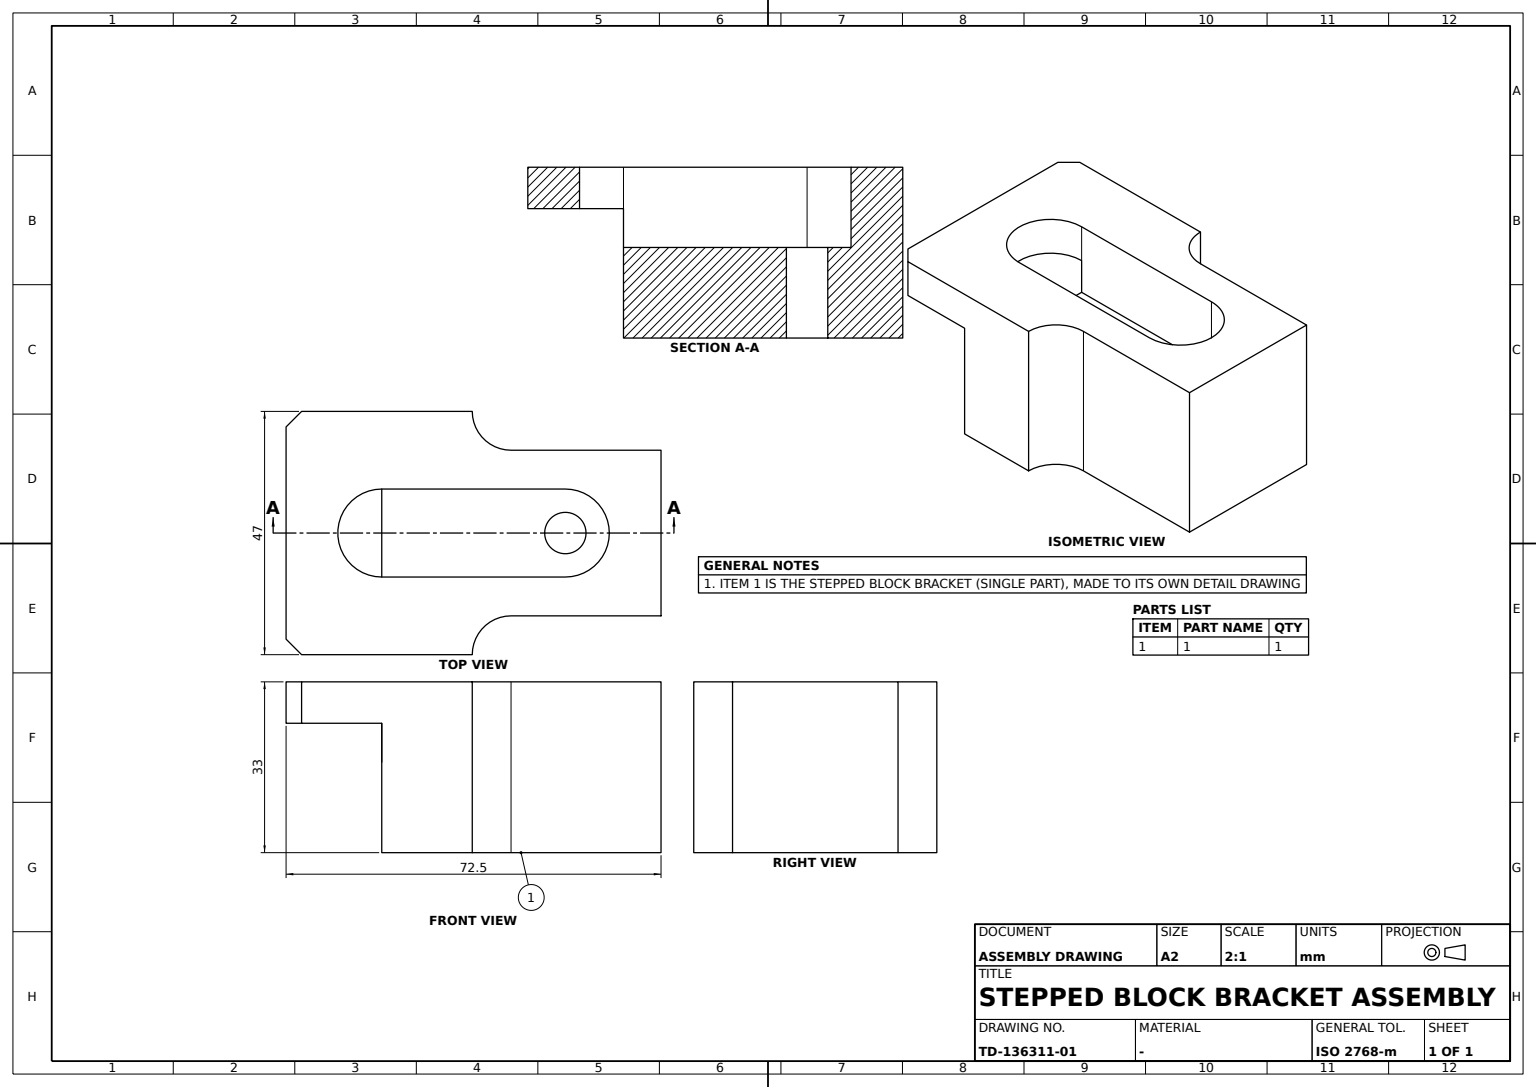
ISO-10303-21;
HEADER;
FILE_DESCRIPTION((''),'2;1');
FILE_NAME('','',(''),(''),'','','');
FILE_SCHEMA(('AUTOMOTIVE_DESIGN'));
ENDSEC;
DATA;
#1=APPLICATION_CONTEXT('');
#2=PRODUCT_CONTEXT('',#1,'mechanical');
#3=PRODUCT('','','',(#2));
#4=PRODUCT_DEFINITION_FORMATION('','',#3);
#5=PRODUCT_DEFINITION_CONTEXT('',#1,'design');
#6=PRODUCT_DEFINITION('','',#4,#5);
#7=PRODUCT_DEFINITION_SHAPE('','',#6);
#8=(LENGTH_UNIT()NAMED_UNIT(*)SI_UNIT(.MILLI.,.METRE.));
#9=(NAMED_UNIT(*)PLANE_ANGLE_UNIT()SI_UNIT($,.RADIAN.));
#10=(NAMED_UNIT(*)SI_UNIT($,.STERADIAN.)SOLID_ANGLE_UNIT());
#11=UNCERTAINTY_MEASURE_WITH_UNIT(LENGTH_MEASURE(1.E-05),#8,'distance_accuracy_value','');
#12=(GEOMETRIC_REPRESENTATION_CONTEXT(3)GLOBAL_UNCERTAINTY_ASSIGNED_CONTEXT((#11))GLOBAL_UNIT_ASSIGNED_CONTEXT((#8,#9,#10))REPRESENTATION_CONTEXT('',''));
#13=CARTESIAN_POINT('',(21.75,0.,17.5));
#14=VERTEX_POINT('',#13);
#15=CARTESIAN_POINT('',(13.75,0.,17.5));
#16=VERTEX_POINT('',#15);
#17=CARTESIAN_POINT('',(17.75,0.,17.5));
#18=DIRECTION('',(0.,0.,1.));
#19=DIRECTION('',(1.,0.,0.));
#20=AXIS2_PLACEMENT_3D('',#17,#18,#19);
#21=CIRCLE('',#20,4.);
#22=EDGE_CURVE('',#14,#16,#21,.T.);
#23=ORIENTED_EDGE('',*,*,#22,.T.);
#24=CARTESIAN_POINT('',(13.75,0.,0.));
#25=VERTEX_POINT('',#24);
#26=CARTESIAN_POINT('',(13.75,0.,-54982.5));
#27=VECTOR('',#18,1000.);
#28=LINE('',#26,#27);
#29=EDGE_CURVE('',#25,#16,#28,.T.);
#30=ORIENTED_EDGE('',*,*,#29,.F.);
#31=CARTESIAN_POINT('',(21.75,0.,0.));
#32=VERTEX_POINT('',#31);
#33=CARTESIAN_POINT('',(17.75,0.,0.));
#34=AXIS2_PLACEMENT_3D('',#33,#18,#19);
#35=CIRCLE('',#34,4.);
#36=EDGE_CURVE('',#32,#25,#35,.T.);
#37=ORIENTED_EDGE('',*,*,#36,.F.);
#38=CARTESIAN_POINT('',(21.75,0.,-54982.5));
#39=LINE('',#38,#27);
#40=EDGE_CURVE('',#32,#14,#39,.T.);
#41=ORIENTED_EDGE('',*,*,#40,.T.);
#42=EDGE_LOOP('',(#23,#30,#37,#41));
#43=FACE_OUTER_BOUND('',#42,.T.);
#44=CARTESIAN_POINT('',(17.75,0.,-54982.5));
#45=AXIS2_PLACEMENT_3D('',#44,#18,#19);
#46=CYLINDRICAL_SURFACE('',#45,4.);
#47=ADVANCED_FACE('',(#43),#46,.F.);
#48=CARTESIAN_POINT('',(-17.75,-8.5,33.));
#49=VERTEX_POINT('',#48);
#50=CARTESIAN_POINT('',(17.75,-8.5,33.));
#51=VERTEX_POINT('',#50);
#52=VECTOR('',#19,1000.);
#53=LINE('',#48,#52);
#54=EDGE_CURVE('',#49,#51,#53,.T.);
#55=ORIENTED_EDGE('',*,*,#54,.F.);
#56=CARTESIAN_POINT('',(-17.75,8.5,33.));
#57=VERTEX_POINT('',#56);
#58=CARTESIAN_POINT('',(-17.75,0.,33.));
#59=AXIS2_PLACEMENT_3D('',#58,#18,#19);
#60=CIRCLE('',#59,8.5);
#61=EDGE_CURVE('',#57,#49,#60,.T.);
#62=ORIENTED_EDGE('',*,*,#61,.F.);
#63=CARTESIAN_POINT('',(17.75,8.5,33.));
#64=VERTEX_POINT('',#63);
#65=DIRECTION('',(-1.,0.,0.));
#66=VECTOR('',#65,1000.);
#67=LINE('',#63,#66);
#68=EDGE_CURVE('',#64,#57,#67,.T.);
#69=ORIENTED_EDGE('',*,*,#68,.F.);
#70=CARTESIAN_POINT('',(26.25,0.,33.));
#71=VERTEX_POINT('',#70);
#72=CARTESIAN_POINT('',(17.75,0.,33.));
#73=AXIS2_PLACEMENT_3D('',#72,#18,#19);
#74=CIRCLE('',#73,8.5);
#75=EDGE_CURVE('',#71,#64,#74,.T.);
#76=ORIENTED_EDGE('',*,*,#75,.F.);
#77=EDGE_CURVE('',#51,#71,#74,.T.);
#78=ORIENTED_EDGE('',*,*,#77,.F.);
#79=EDGE_LOOP('',(#55,#62,#69,#76,#78));
#80=FACE_BOUND('',#79,.T.);
#81=CARTESIAN_POINT('',(36.25,-16.,33.));
#82=VERTEX_POINT('',#81);
#83=CARTESIAN_POINT('',(7.25,-16.,33.));
#84=VERTEX_POINT('',#83);
#85=LINE('',#81,#66);
#86=EDGE_CURVE('',#82,#84,#85,.T.);
#87=ORIENTED_EDGE('',*,*,#86,.F.);
#88=CARTESIAN_POINT('',(36.25,16.,33.));
#89=VERTEX_POINT('',#88);
#90=CARTESIAN_POINT('',(36.25,-23.5,33.));
#91=DIRECTION('',(0.,1.,0.));
#92=VECTOR('',#91,1000.);
#93=LINE('',#90,#92);
#94=EDGE_CURVE('',#82,#89,#93,.T.);
#95=ORIENTED_EDGE('',*,*,#94,.T.);
#96=CARTESIAN_POINT('',(7.25,16.,33.));
#97=VERTEX_POINT('',#96);
#98=CARTESIAN_POINT('',(-0.25,16.,33.));
#99=LINE('',#98,#52);
#100=EDGE_CURVE('',#97,#89,#99,.T.);
#101=ORIENTED_EDGE('',*,*,#100,.F.);
#102=CARTESIAN_POINT('',(-0.25,23.5,33.));
#103=VERTEX_POINT('',#102);
#104=CARTESIAN_POINT('',(7.25,23.5,33.));
#105=DIRECTION('',(0.,0.,-1.));
#106=AXIS2_PLACEMENT_3D('',#104,#105,#19);
#107=CIRCLE('',#106,7.5);
#108=EDGE_CURVE('',#97,#103,#107,.T.);
#109=ORIENTED_EDGE('',*,*,#108,.T.);
#110=CARTESIAN_POINT('',(-33.25,23.5,33.));
#111=VERTEX_POINT('',#110);
#112=CARTESIAN_POINT('',(36.25,23.5,33.));
#113=LINE('',#112,#66);
#114=EDGE_CURVE('',#103,#111,#113,.T.);
#115=ORIENTED_EDGE('',*,*,#114,.T.);
#116=CARTESIAN_POINT('',(-36.25,20.5,33.));
#117=VERTEX_POINT('',#116);
#118=DIRECTION('',(-0.707106781,-0.707106781,0.));
#119=VECTOR('',#118,1000.);
#120=LINE('',#110,#119);
#121=EDGE_CURVE('',#111,#117,#120,.T.);
#122=ORIENTED_EDGE('',*,*,#121,.T.);
#123=CARTESIAN_POINT('',(-36.25,-20.5,33.));
#124=VERTEX_POINT('',#123);
#125=DIRECTION('',(0.,-1.,0.));
#126=VECTOR('',#125,1000.);
#127=LINE('',#116,#126);
#128=EDGE_CURVE('',#117,#124,#127,.T.);
#129=ORIENTED_EDGE('',*,*,#128,.T.);
#130=CARTESIAN_POINT('',(-33.25,-23.5,33.));
#131=VERTEX_POINT('',#130);
#132=DIRECTION('',(0.707106781,-0.707106781,0.));
#133=VECTOR('',#132,1000.);
#134=LINE('',#123,#133);
#135=EDGE_CURVE('',#124,#131,#134,.T.);
#136=ORIENTED_EDGE('',*,*,#135,.T.);
#137=CARTESIAN_POINT('',(-0.25,-23.5,33.));
#138=VERTEX_POINT('',#137);
#139=LINE('',#130,#52);
#140=EDGE_CURVE('',#131,#138,#139,.T.);
#141=ORIENTED_EDGE('',*,*,#140,.T.);
#142=CARTESIAN_POINT('',(7.25,-23.5,33.));
#143=AXIS2_PLACEMENT_3D('',#142,#105,#19);
#144=CIRCLE('',#143,7.5);
#145=EDGE_CURVE('',#138,#84,#144,.T.);
#146=ORIENTED_EDGE('',*,*,#145,.T.);
#147=EDGE_LOOP('',(#87,#95,#101,#109,#115,#122,#129,#136,#141,#146));
#148=FACE_OUTER_BOUND('',#147,.T.);
#149=CARTESIAN_POINT('',(0.,0.,33.));
#150=AXIS2_PLACEMENT_3D('',#149,#18,#19);
#151=PLANE('',#150);
#152=ADVANCED_FACE('',(#80,#148),#151,.T.);
#153=CARTESIAN_POINT('',(-17.75,-8.5,25.));
#154=VERTEX_POINT('',#153);
#155=CARTESIAN_POINT('',(-17.75,-8.5,17.5));
#156=VECTOR('',#105,1000.);
#157=LINE('',#155,#156);
#158=EDGE_CURVE('',#49,#154,#157,.T.);
#159=ORIENTED_EDGE('',*,*,#158,.T.);
#160=CARTESIAN_POINT('',(-17.75,8.5,25.));
#161=VERTEX_POINT('',#160);
#162=CARTESIAN_POINT('',(-17.75,0.,25.));
#163=AXIS2_PLACEMENT_3D('',#162,#18,#19);
#164=CIRCLE('',#163,8.5);
#165=EDGE_CURVE('',#161,#154,#164,.T.);
#166=ORIENTED_EDGE('',*,*,#165,.F.);
#167=CARTESIAN_POINT('',(-17.75,8.5,17.5));
#168=LINE('',#167,#156);
#169=EDGE_CURVE('',#57,#161,#168,.T.);
#170=ORIENTED_EDGE('',*,*,#169,.F.);
#171=ORIENTED_EDGE('',*,*,#61,.T.);
#172=EDGE_LOOP('',(#159,#166,#170,#171));
#173=FACE_OUTER_BOUND('',#172,.T.);
#174=CARTESIAN_POINT('',(-17.75,0.,17.5));
#175=AXIS2_PLACEMENT_3D('',#174,#18,#19);
#176=CYLINDRICAL_SURFACE('',#175,8.5);
#177=ADVANCED_FACE('',(#173),#176,.F.);
#178=CARTESIAN_POINT('',(-36.25,-20.5,25.));
#179=VERTEX_POINT('',#178);
#180=LINE('',#123,#156);
#181=EDGE_CURVE('',#124,#179,#180,.T.);
#182=ORIENTED_EDGE('',*,*,#181,.F.);
#183=ORIENTED_EDGE('',*,*,#128,.F.);
#184=CARTESIAN_POINT('',(-36.25,20.5,25.));
#185=VERTEX_POINT('',#184);
#186=LINE('',#116,#156);
#187=EDGE_CURVE('',#117,#185,#186,.T.);
#188=ORIENTED_EDGE('',*,*,#187,.T.);
#189=CARTESIAN_POINT('',(-36.25,54976.5,25.));
#190=LINE('',#189,#126);
#191=EDGE_CURVE('',#185,#179,#190,.T.);
#192=ORIENTED_EDGE('',*,*,#191,.T.);
#193=EDGE_LOOP('',(#182,#183,#188,#192));
#194=FACE_OUTER_BOUND('',#193,.T.);
#195=AXIS2_PLACEMENT_3D('',#116,#19,#91);
#196=PLANE('',#195);
#197=ADVANCED_FACE('',(#194),#196,.F.);
#198=CARTESIAN_POINT('',(-0.25,-23.5,0.));
#199=VERTEX_POINT('',#198);
#200=LINE('',#198,#27);
#201=EDGE_CURVE('',#199,#138,#200,.T.);
#202=ORIENTED_EDGE('',*,*,#201,.T.);
#203=ORIENTED_EDGE('',*,*,#140,.F.);
#204=CARTESIAN_POINT('',(-33.25,-23.5,25.));
#205=VERTEX_POINT('',#204);
#206=LINE('',#130,#156);
#207=EDGE_CURVE('',#131,#205,#206,.T.);
#208=ORIENTED_EDGE('',*,*,#207,.T.);
#209=CARTESIAN_POINT('',(-17.75,-23.5,25.));
#210=VERTEX_POINT('',#209);
#211=LINE('',#209,#66);
#212=EDGE_CURVE('',#210,#205,#211,.T.);
#213=ORIENTED_EDGE('',*,*,#212,.F.);
#214=CARTESIAN_POINT('',(-17.75,-23.5,0.));
#215=VERTEX_POINT('',#214);
#216=LINE('',#214,#27);
#217=EDGE_CURVE('',#215,#210,#216,.T.);
#218=ORIENTED_EDGE('',*,*,#217,.F.);
#219=CARTESIAN_POINT('',(-33.25,-23.5,0.));
#220=LINE('',#219,#52);
#221=EDGE_CURVE('',#215,#199,#220,.T.);
#222=ORIENTED_EDGE('',*,*,#221,.T.);
#223=EDGE_LOOP('',(#202,#203,#208,#213,#218,#222));
#224=FACE_OUTER_BOUND('',#223,.T.);
#225=AXIS2_PLACEMENT_3D('',#130,#91,#18);
#226=PLANE('',#225);
#227=ADVANCED_FACE('',(#224),#226,.F.);
#228=ORIENTED_EDGE('',*,*,#121,.F.);
#229=CARTESIAN_POINT('',(-33.25,23.5,25.));
#230=VERTEX_POINT('',#229);
#231=LINE('',#110,#156);
#232=EDGE_CURVE('',#111,#230,#231,.T.);
#233=ORIENTED_EDGE('',*,*,#232,.T.);
#234=LINE('',#229,#119);
#235=EDGE_CURVE('',#230,#185,#234,.T.);
#236=ORIENTED_EDGE('',*,*,#235,.T.);
#237=ORIENTED_EDGE('',*,*,#187,.F.);
#238=EDGE_LOOP('',(#228,#233,#236,#237));
#239=FACE_OUTER_BOUND('',#238,.T.);
#240=DIRECTION('',(0.707106781,0.707106781,0.));
#241=AXIS2_PLACEMENT_3D('',#110,#132,#240);
#242=PLANE('',#241);
#243=ADVANCED_FACE('',(#239),#242,.F.);
#244=CARTESIAN_POINT('',(36.25,16.,0.));
#245=VERTEX_POINT('',#244);
#246=CARTESIAN_POINT('',(36.25,16.,-54967.));
#247=LINE('',#246,#27);
#248=EDGE_CURVE('',#245,#89,#247,.T.);
#249=ORIENTED_EDGE('',*,*,#248,.T.);
#250=ORIENTED_EDGE('',*,*,#94,.F.);
#251=CARTESIAN_POINT('',(36.25,-16.,0.));
#252=VERTEX_POINT('',#251);
#253=LINE('',#251,#27);
#254=EDGE_CURVE('',#252,#82,#253,.T.);
#255=ORIENTED_EDGE('',*,*,#254,.F.);
#256=CARTESIAN_POINT('',(36.25,-23.5,0.));
#257=LINE('',#256,#92);
#258=EDGE_CURVE('',#252,#245,#257,.T.);
#259=ORIENTED_EDGE('',*,*,#258,.T.);
#260=EDGE_LOOP('',(#249,#250,#255,#259));
#261=FACE_OUTER_BOUND('',#260,.T.);
#262=AXIS2_PLACEMENT_3D('',#90,#65,#125);
#263=PLANE('',#262);
#264=ADVANCED_FACE('',(#261),#263,.F.);
#265=CARTESIAN_POINT('',(7.25,-16.,0.));
#266=VERTEX_POINT('',#265);
#267=CARTESIAN_POINT('',(7.25,-23.5,0.));
#268=AXIS2_PLACEMENT_3D('',#267,#18,#19);
#269=CIRCLE('',#268,7.5);
#270=EDGE_CURVE('',#266,#199,#269,.T.);
#271=ORIENTED_EDGE('',*,*,#270,.F.);
#272=LINE('',#265,#156);
#273=EDGE_CURVE('',#84,#266,#272,.T.);
#274=ORIENTED_EDGE('',*,*,#273,.F.);
#275=ORIENTED_EDGE('',*,*,#145,.F.);
#276=ORIENTED_EDGE('',*,*,#201,.F.);
#277=EDGE_LOOP('',(#271,#274,#275,#276));
#278=FACE_OUTER_BOUND('',#277,.T.);
#279=CYLINDRICAL_SURFACE('',#268,7.5);
#280=ADVANCED_FACE('',(#278),#279,.F.);
#281=ORIENTED_EDGE('',*,*,#77,.T.);
#282=CARTESIAN_POINT('',(26.25,0.,17.5));
#283=VERTEX_POINT('',#282);
#284=LINE('',#282,#27);
#285=EDGE_CURVE('',#283,#71,#284,.T.);
#286=ORIENTED_EDGE('',*,*,#285,.F.);
#287=CARTESIAN_POINT('',(17.75,-8.5,17.5));
#288=VERTEX_POINT('',#287);
#289=AXIS2_PLACEMENT_3D('',#17,#105,#19);
#290=CIRCLE('',#289,8.5);
#291=EDGE_CURVE('',#283,#288,#290,.T.);
#292=ORIENTED_EDGE('',*,*,#291,.T.);
#293=LINE('',#287,#156);
#294=EDGE_CURVE('',#51,#288,#293,.T.);
#295=ORIENTED_EDGE('',*,*,#294,.F.);
#296=EDGE_LOOP('',(#281,#286,#292,#295));
#297=FACE_OUTER_BOUND('',#296,.T.);
#298=CYLINDRICAL_SURFACE('',#20,8.5);
#299=ADVANCED_FACE('',(#297),#298,.F.);
#300=EDGE_CURVE('',#25,#32,#35,.T.);
#301=ORIENTED_EDGE('',*,*,#300,.F.);
#302=ORIENTED_EDGE('',*,*,#29,.T.);
#303=EDGE_CURVE('',#16,#14,#21,.T.);
#304=ORIENTED_EDGE('',*,*,#303,.T.);
#305=ORIENTED_EDGE('',*,*,#40,.F.);
#306=EDGE_LOOP('',(#301,#302,#304,#305));
#307=FACE_OUTER_BOUND('',#306,.T.);
#308=ADVANCED_FACE('',(#307),#46,.F.);
#309=ORIENTED_EDGE('',*,*,#258,.F.);
#310=LINE('',#251,#66);
#311=EDGE_CURVE('',#252,#266,#310,.T.);
#312=ORIENTED_EDGE('',*,*,#311,.T.);
#313=ORIENTED_EDGE('',*,*,#270,.T.);
#314=ORIENTED_EDGE('',*,*,#221,.F.);
#315=CARTESIAN_POINT('',(-17.75,23.5,0.));
#316=VERTEX_POINT('',#315);
#317=CARTESIAN_POINT('',(-17.75,54976.5,0.));
#318=LINE('',#317,#126);
#319=EDGE_CURVE('',#316,#215,#318,.T.);
#320=ORIENTED_EDGE('',*,*,#319,.F.);
#321=CARTESIAN_POINT('',(-0.25,23.5,0.));
#322=VERTEX_POINT('',#321);
#323=CARTESIAN_POINT('',(36.25,23.5,0.));
#324=LINE('',#323,#66);
#325=EDGE_CURVE('',#322,#316,#324,.T.);
#326=ORIENTED_EDGE('',*,*,#325,.F.);
#327=CARTESIAN_POINT('',(7.25,16.,0.));
#328=VERTEX_POINT('',#327);
#329=CARTESIAN_POINT('',(7.25,23.5,0.));
#330=AXIS2_PLACEMENT_3D('',#329,#18,#19);
#331=CIRCLE('',#330,7.5);
#332=EDGE_CURVE('',#322,#328,#331,.T.);
#333=ORIENTED_EDGE('',*,*,#332,.T.);
#334=CARTESIAN_POINT('',(0.,16.,0.));
#335=LINE('',#334,#52);
#336=EDGE_CURVE('',#328,#245,#335,.T.);
#337=ORIENTED_EDGE('',*,*,#336,.T.);
#338=EDGE_LOOP('',(#309,#312,#313,#314,#320,#326,#333,#337));
#339=FACE_OUTER_BOUND('',#338,.T.);
#340=ORIENTED_EDGE('',*,*,#300,.T.);
#341=ORIENTED_EDGE('',*,*,#36,.T.);
#342=EDGE_LOOP('',(#340,#341));
#343=FACE_BOUND('',#342,.T.);
#344=CARTESIAN_POINT('',(0.,0.,0.));
#345=AXIS2_PLACEMENT_3D('',#344,#18,#19);
#346=PLANE('',#345);
#347=ADVANCED_FACE('',(#339,#343),#346,.F.);
#348=ORIENTED_EDGE('',*,*,#212,.T.);
#349=LINE('',#178,#133);
#350=EDGE_CURVE('',#179,#205,#349,.T.);
#351=ORIENTED_EDGE('',*,*,#350,.F.);
#352=ORIENTED_EDGE('',*,*,#191,.F.);
#353=ORIENTED_EDGE('',*,*,#235,.F.);
#354=CARTESIAN_POINT('',(-17.75,23.5,25.));
#355=VERTEX_POINT('',#354);
#356=CARTESIAN_POINT('',(36.25,23.5,25.));
#357=LINE('',#356,#66);
#358=EDGE_CURVE('',#355,#230,#357,.T.);
#359=ORIENTED_EDGE('',*,*,#358,.F.);
#360=CARTESIAN_POINT('',(-17.75,54976.5,25.));
#361=LINE('',#360,#92);
#362=EDGE_CURVE('',#161,#355,#361,.T.);
#363=ORIENTED_EDGE('',*,*,#362,.F.);
#364=ORIENTED_EDGE('',*,*,#165,.T.);
#365=EDGE_CURVE('',#210,#154,#361,.T.);
#366=ORIENTED_EDGE('',*,*,#365,.F.);
#367=EDGE_LOOP('',(#348,#351,#352,#353,#359,#363,#364,#366));
#368=FACE_OUTER_BOUND('',#367,.T.);
#369=AXIS2_PLACEMENT_3D('',#360,#18,#19);
#370=PLANE('',#369);
#371=ADVANCED_FACE('',(#368),#370,.F.);
#372=ORIENTED_EDGE('',*,*,#108,.F.);
#373=LINE('',#96,#27);
#374=EDGE_CURVE('',#328,#97,#373,.T.);
#375=ORIENTED_EDGE('',*,*,#374,.F.);
#376=ORIENTED_EDGE('',*,*,#332,.F.);
#377=CARTESIAN_POINT('',(-0.25,23.5,-54967.));
#378=LINE('',#377,#27);
#379=EDGE_CURVE('',#322,#103,#378,.T.);
#380=ORIENTED_EDGE('',*,*,#379,.T.);
#381=EDGE_LOOP('',(#372,#375,#376,#380));
#382=FACE_OUTER_BOUND('',#381,.T.);
#383=CARTESIAN_POINT('',(7.25,23.5,-54967.));
#384=AXIS2_PLACEMENT_3D('',#383,#18,#19);
#385=CYLINDRICAL_SURFACE('',#384,7.5);
#386=ADVANCED_FACE('',(#382),#385,.F.);
#387=ORIENTED_EDGE('',*,*,#365,.T.);
#388=VERTEX_POINT('',#155);
#389=LINE('',#155,#27);
#390=EDGE_CURVE('',#388,#154,#389,.T.);
#391=ORIENTED_EDGE('',*,*,#390,.F.);
#392=VERTEX_POINT('',#167);
#393=CARTESIAN_POINT('',(-17.75,54976.5,17.5));
#394=LINE('',#393,#126);
#395=EDGE_CURVE('',#392,#388,#394,.T.);
#396=ORIENTED_EDGE('',*,*,#395,.F.);
#397=LINE('',#167,#27);
#398=EDGE_CURVE('',#392,#161,#397,.T.);
#399=ORIENTED_EDGE('',*,*,#398,.T.);
#400=ORIENTED_EDGE('',*,*,#362,.T.);
#401=CARTESIAN_POINT('',(-17.75,23.5,33.));
#402=LINE('',#401,#27);
#403=EDGE_CURVE('',#316,#355,#402,.T.);
#404=ORIENTED_EDGE('',*,*,#403,.F.);
#405=ORIENTED_EDGE('',*,*,#319,.T.);
#406=ORIENTED_EDGE('',*,*,#217,.T.);
#407=EDGE_LOOP('',(#387,#391,#396,#399,#400,#404,#405,#406));
#408=FACE_OUTER_BOUND('',#407,.T.);
#409=AXIS2_PLACEMENT_3D('',#317,#19,#105);
#410=PLANE('',#409);
#411=ADVANCED_FACE('',(#408),#410,.F.);
#412=CARTESIAN_POINT('',(17.75,8.5,17.5));
#413=VERTEX_POINT('',#412);
#414=EDGE_CURVE('',#413,#283,#290,.T.);
#415=ORIENTED_EDGE('',*,*,#414,.T.);
#416=ORIENTED_EDGE('',*,*,#285,.T.);
#417=ORIENTED_EDGE('',*,*,#75,.T.);
#418=LINE('',#412,#156);
#419=EDGE_CURVE('',#64,#413,#418,.T.);
#420=ORIENTED_EDGE('',*,*,#419,.T.);
#421=EDGE_LOOP('',(#415,#416,#417,#420));
#422=FACE_OUTER_BOUND('',#421,.T.);
#423=ADVANCED_FACE('',(#422),#298,.F.);
#424=ORIENTED_EDGE('',*,*,#114,.F.);
#425=ORIENTED_EDGE('',*,*,#379,.F.);
#426=ORIENTED_EDGE('',*,*,#325,.T.);
#427=ORIENTED_EDGE('',*,*,#403,.T.);
#428=ORIENTED_EDGE('',*,*,#358,.T.);
#429=ORIENTED_EDGE('',*,*,#232,.F.);
#430=EDGE_LOOP('',(#424,#425,#426,#427,#428,#429));
#431=FACE_OUTER_BOUND('',#430,.T.);
#432=AXIS2_PLACEMENT_3D('',#112,#125,#105);
#433=PLANE('',#432);
#434=ADVANCED_FACE('',(#431),#433,.F.);
#435=ORIENTED_EDGE('',*,*,#100,.T.);
#436=ORIENTED_EDGE('',*,*,#248,.F.);
#437=ORIENTED_EDGE('',*,*,#336,.F.);
#438=ORIENTED_EDGE('',*,*,#374,.T.);
#439=EDGE_LOOP('',(#435,#436,#437,#438));
#440=FACE_OUTER_BOUND('',#439,.T.);
#441=CARTESIAN_POINT('',(-0.25,16.,-54967.));
#442=AXIS2_PLACEMENT_3D('',#441,#125,#105);
#443=PLANE('',#442);
#444=ADVANCED_FACE('',(#440),#443,.F.);
#445=ORIENTED_EDGE('',*,*,#350,.T.);
#446=ORIENTED_EDGE('',*,*,#207,.F.);
#447=ORIENTED_EDGE('',*,*,#135,.F.);
#448=ORIENTED_EDGE('',*,*,#181,.T.);
#449=EDGE_LOOP('',(#445,#446,#447,#448));
#450=FACE_OUTER_BOUND('',#449,.T.);
#451=DIRECTION('',(-0.707106781,0.707106781,0.));
#452=AXIS2_PLACEMENT_3D('',#123,#240,#451);
#453=PLANE('',#452);
#454=ADVANCED_FACE('',(#450),#453,.F.);
#455=LINE('',#155,#66);
#456=EDGE_CURVE('',#288,#388,#455,.T.);
#457=ORIENTED_EDGE('',*,*,#456,.T.);
#458=ORIENTED_EDGE('',*,*,#390,.T.);
#459=ORIENTED_EDGE('',*,*,#158,.F.);
#460=ORIENTED_EDGE('',*,*,#54,.T.);
#461=ORIENTED_EDGE('',*,*,#294,.T.);
#462=EDGE_LOOP('',(#457,#458,#459,#460,#461));
#463=FACE_OUTER_BOUND('',#462,.T.);
#464=AXIS2_PLACEMENT_3D('',#155,#125,#105);
#465=PLANE('',#464);
#466=ADVANCED_FACE('',(#463),#465,.F.);
#467=ORIENTED_EDGE('',*,*,#311,.F.);
#468=ORIENTED_EDGE('',*,*,#254,.T.);
#469=ORIENTED_EDGE('',*,*,#86,.T.);
#470=ORIENTED_EDGE('',*,*,#273,.T.);
#471=EDGE_LOOP('',(#467,#468,#469,#470));
#472=FACE_OUTER_BOUND('',#471,.T.);
#473=AXIS2_PLACEMENT_3D('',#251,#91,#18);
#474=PLANE('',#473);
#475=ADVANCED_FACE('',(#472),#474,.F.);
#476=ORIENTED_EDGE('',*,*,#395,.T.);
#477=ORIENTED_EDGE('',*,*,#456,.F.);
#478=ORIENTED_EDGE('',*,*,#291,.F.);
#479=ORIENTED_EDGE('',*,*,#414,.F.);
#480=LINE('',#412,#52);
#481=EDGE_CURVE('',#392,#413,#480,.T.);
#482=ORIENTED_EDGE('',*,*,#481,.F.);
#483=EDGE_LOOP('',(#476,#477,#478,#479,#482));
#484=FACE_OUTER_BOUND('',#483,.T.);
#485=ORIENTED_EDGE('',*,*,#303,.F.);
#486=ORIENTED_EDGE('',*,*,#22,.F.);
#487=EDGE_LOOP('',(#485,#486));
#488=FACE_BOUND('',#487,.T.);
#489=PLANE('',#175);
#490=ADVANCED_FACE('',(#484,#488),#489,.T.);
#491=ORIENTED_EDGE('',*,*,#481,.T.);
#492=ORIENTED_EDGE('',*,*,#419,.F.);
#493=ORIENTED_EDGE('',*,*,#68,.T.);
#494=ORIENTED_EDGE('',*,*,#169,.T.);
#495=ORIENTED_EDGE('',*,*,#398,.F.);
#496=EDGE_LOOP('',(#491,#492,#493,#494,#495));
#497=FACE_OUTER_BOUND('',#496,.T.);
#498=AXIS2_PLACEMENT_3D('',#412,#91,#18);
#499=PLANE('',#498);
#500=ADVANCED_FACE('',(#497),#499,.F.);
#501=CLOSED_SHELL('',(#47,#152,#177,#197,#227,#243,#264,#280,#299,#308,#347,#371,#386,#411,#423,#434,#444,#454,#466,#475,#490,#500));
#502=MANIFOLD_SOLID_BREP('',#501);
#503=ADVANCED_BREP_SHAPE_REPRESENTATION('',(#502),#12);
#504=SHAPE_DEFINITION_REPRESENTATION(#7,#503);
ENDSEC;
END-ISO-10303-21;
